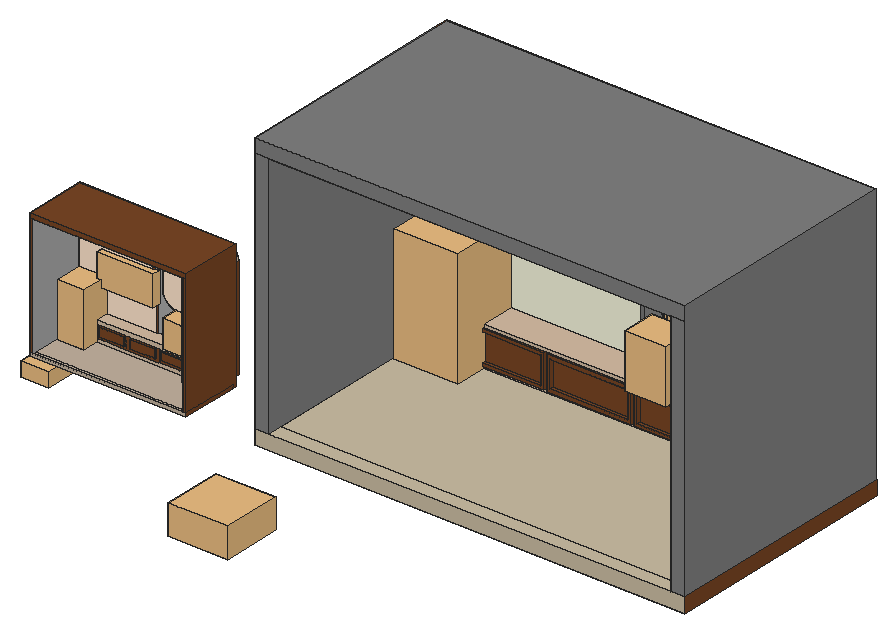
# SketchUp Ruby script. Lengths in inches.
U = 1.inch
M = Sketchup.active_model
def pt(a) = Geom::Point3d.new(a.map { |v| v * U })
def face(e, loops, mat)
  f = e.add_face(loops[0].map { |a| pt(a) })
  loops[1..].each { |l| e.add_face(l.map { |a| pt(a) }).erase! }
  f.material = f.back_material = mat if mat
  f
end
# faces: each face lists its corners as indices into pts; further lists are holes
def faces(e, pts, list, mat = nil) = list.each { |f| face(e, (f[0].is_a?(Array) ? f : [f]).map { |l| l.map { |i| pts[i] } }, mat) }
# xy, xz, yz: faces in a plane at the given z, y or x. An outline is a flat list of corners, or four numbers for a rectangle; further outlines are holes
def ring(l) = l.size == 4 ? [[l[0], l[1]], [l[2], l[1]], [l[2], l[3]], [l[0], l[3]]] : l.each_slice(2).to_a
def flat(e, list, mat, &to3) = list.each { |f| face(e, (f[0].is_a?(Array) ? f : [f]).map { |l| ring(l).map { |u, v| to3.(u, v) } }, mat) }
def xy(e, z, list, mat = nil) = flat(e, list, mat) { |x, y| [x, y, z] }
def xz(e, y, list, mat = nil) = flat(e, list, mat) { |x, z| [x, y, z] }
def yz(e, x, list, mat = nil) = flat(e, list, mat) { |y, z| [x, y, z] }
def lines(e, pts, list) = list.each { |a, b| e.add_line(pt(pts[a]), pt(pts[b])) }
# prism: a flat outline (further loops are holes) pulled along v
def prism(e, loops, v, mat = nil)
  f = face(e, loops, mat); d = Geom::Vector3d.new(v.map { |x| x * U })
  f.pushpull(f.normal.samedirection?(d) ? d.length : -d.length)
end
def box(e, o, s, mat = nil) = prism(e, [[o, [o[0] + s[0], o[1], o[2]], [o[0] + s[0], o[1] + s[1], o[2]], [o[0], o[1] + s[1], o[2]]]], [0, 0, s[2]], mat)
def at(x, y, z, deg = 0) = Geom::Transformation.translation(pt([x, y, z])) * Geom::Transformation.rotation(ORIGIN, Z_AXIS, deg.degrees)
def axes(o, x, y, z) = Geom::Transformation.new([*x, 0, *y, 0, *z, 0, *pt(o).to_a, 1])
def part(name) = M.definitions.add(name)
# library, detail: a bought-in or finely detailed component or shape, given as its bounding box
def library(name, o, s) = part(name).tap { |d| box(d.entities, o, s) }
def detail(e, o, s) = box(e.add_group.entities, o, s)
def put(e, d, t, mat = nil) = e.add_instance(d, t).tap { |i| i.material = mat if mat }
def group(e, t, mat = nil) = e.add_group.tap { |g| g.transformation = t; g.material = mat if mat }.entities
root = M.entities
M.materials.add("[0049_Beige]").color = [245, 245, 220]
M.materials.add("[0131_Silver]").color = [192, 192, 192]
M.materials.add("[0132_LightGray]").color = [169, 169, 169]
M.materials.add("[0133_Gray]").color = [128, 128, 128]
M.materials.add("[Color C01]").color = [255, 229, 204]
M.materials.add("[Concrete Tile]").color = [203, 190, 164]
M.materials.add("[Formica Laminate Light]").color = [213, 189, 164]
M.materials.add("[Tile Large Brown]").color = [195, 178, 159]
M.materials.add("[Wood Veneer 01]").color = [120, 70, 37]
c1 = library("Vase 296 007 001",[-21.53,-18.1,-0.16],[43.06,36.19,57.09])
c2 = library("False Aralia 002",[-20.33,-19.19,0],[40.48,38.23,49.87])
c3 = library("Clock Wall 005",[-16.6,-6.65,-37.13],[33.15,6.65,38.31])
c4 = library("Television screen",[0,1.41,1.14],[35.92,0.28,20.21])
c5 = library("Spot Light",[-5.1,-5.1,-11.05],[10.2,10.2,11.05])
c6 = library("Dome Light",[-12,-12,0],[24,24,12])
c7 = part("Group16\#1")
p = [[0,0,0],[0,0,-66.45],[-11.6,0,-66.45],[75.53,-139.58,0],[-75.53,-139.58,0],[75.53,139.58,0],
  [75.53,0,0],[-75.53,139.58,0],[11.6,0,-66.45],[-75.53,0,0],[0,0,-107.56]]
lines(c7.entities,p,[[0,1],[1,2],[3,4],[5,6],[7,5],[1,8],[9,0],[0,6],[8,10],[4,9],[6,3],[2,10],
  [9,7]])
c8 = part("Rectangle Light")
put(c8.entities,c7,at(0,0,0))
c9 = library("Omni Light",[-12,-12,-12],[24,24,24])
c10 = library("Omni Light\#1",[-12,-12,-12],[24,24,24])
c11 = library("Omni Light\#2",[-12,-12,-12],[24,24,24])
c12 = library("Omni Light\#3",[-12,-12,-12],[24,24,24])
c13 = library("Omni Light\#4",[-12,-12,-12],[24,24,24])
c14 = library("Omni Light\#5",[-12,-12,-12],[24,24,24])
c15 = library("Omni Light\#6",[-12,-12,-12],[24,24,24])
c16 = library("Omni Light\#7",[-12,-12,-12],[24,24,24])
c17 = library("Omni Light\#8",[-12,-12,-12],[24,24,24])
c18 = library("Omni Light\#9",[-12,-12,-12],[24,24,24])
c19 = library("Omni Light\#10",[-12,-12,-12],[24,24,24])
c20 = library("Omni Light\#11",[-12,-12,-12],[24,24,24])
c21 = library("Omni Light\#12",[-12,-12,-12],[24,24,24])
c22 = library("Omni Light\#13",[-12,-12,-12],[24,24,24])
c23 = library("Omni Light\#14",[-12,-12,-12],[24,24,24])
c24 = library("Omni Light\#15",[-12,-12,-12],[24,24,24])
c25 = library("Omni Light\#16",[-12,-12,-12],[24,24,24])
c26 = library("Omni Light\#17",[-12,-12,-12],[24,24,24])
c27 = library("Omni Light\#18",[-12,-12,-12],[24,24,24])
c28 = library("Omni Light\#19",[-12,-12,-12],[24,24,24])
c29 = library("Omni Light\#20",[-12,-12,-12],[24,24,24])
c30 = library("Omni Light\#21",[-12,-12,-12],[24,24,24])
c31 = library("Omni Light\#22",[-12,-12,-12],[24,24,24])
c32 = library("Omni Light\#23",[-12,-12,-12],[24,24,24])
c33 = library("Omni Light\#24",[-12,-12,-12],[24,24,24])
c34 = library("Omni Light\#25",[-12,-12,-12],[24,24,24])
c35 = library("Dome Light\#1",[-12,-12,0],[24,24,12])
c36 = library("Group\#5",[0,0,0],[151,81.0625,281.6875])
c37 = library("Group\#7",[0,0,0],[106.53,4.9375,165.91])
xy(root,0,[[472.95,0,1373.83,501.25]],"[Wood Veneer 01]")
xy(root,7.3125,[[7.02,1.49,320.41,8.52],[7.02,8.52,320.41,8.52,320.41,78.66,314.79,78.66,314.79,154.47,262.16,154.47,262.16,78.66,256.35,78.66,256.35,124.34,256.15,124.34,256.15,95.03,64.79,95.03,63.9,95.09,63.02,95.26,62.18,95.55,61.375,95.95,60.63,96.44,59.96,97.03,59.37,97.7,58.875,98.45,58.48,99.25,58.19,100.09,58.02,100.97,57.96,101.86,57.96,121.47,7.02,121.47]],"[Tile Large Brown]")
xy(root,19.25,[[68.6,95.03,122.4,97.28],[134.41,95.03,188.21,97.28],[199.24,95.03,253.04,97.28]],"[Wood Veneer 01]")
xy(root,19.89,[[199.875,95.03,252.4,97.28]],"[Wood Veneer 01]")
xy(root,20.02,[[135.18,95.03,187.44,97.28]],"[Wood Veneer 01]")
xy(root,20.04,[[69.39,95.03,121.61,97.28]],"[Wood Veneer 01]")
xy(root,30.1875,[[472.95,0,1373.83,0,1373.83,471.59,1344.17,471.59,1344.17,29.66,502.62,29.66,502.62,471.59,472.95,471.59],[502.62,29.66,1344.17,29.66,1344.17,471.59,1342.17,471.59,1342.17,390.53,1323.54,390.53,1323.54,471.59,1312.73,471.59,1312.73,390.53,1306.5,390.53,1306.5,471.59,1295.58,471.59,1295.58,386.34,1290.74,386.34,1290.74,471.59,1183.92,471.59,1183.92,386.34,1179.08,386.34,1179.08,471.59,1168.14,471.59,1168.14,390.53,1161.92,390.53,1161.92,471.59,1147.79,471.59,1147.79,390.53,1126.36,390.53,1126.36,392.15,599.34,392.15,599.34,471.59,502.62,471.59]],"[Concrete Tile]")
xy(root,30.1875,[[599.34,392.15,1126.36,471.59]],"[Wood Veneer 01]")
xy(root,36.08,[[605.24,387.03,768.36,392.15],[774.36,387.03,951.86,392.15],[957.86,387.03,1120.46,392.15]],"[Wood Veneer 01]")
xy(root,37.21,[[69.39,95.03,121.61,97.28]],"[Wood Veneer 01]")
xy(root,37.23,[[135.18,95.03,187.44,97.28]],"[Wood Veneer 01]")
xy(root,37.36,[[199.875,95.03,252.4,97.28]],"[Wood Veneer 01]")
xy(root,38,[[68.6,95.03,122.4,97.28],[134.41,95.03,188.21,97.28],[199.24,95.03,253.04,97.28]],"[Wood Veneer 01]")
xy(root,41.83,[[610.98,387.03,762.62,395.59]],"[Wood Veneer 01]")
xy(root,42.55,[[964.33,387.03,1113.99,394.15]],"[Wood Veneer 01]")
xy(root,43.18,[[781.45,387.03,944.77,394.15]],"[Wood Veneer 01]")
xy(root,50.1875,[[64.79,95.03,65.54,95.03,65.54,95.87,64.65,95.92,63.78,96.1,62.93,96.38,62.13,96.78,61.39,97.28,60.72,97.86,60.13,98.54,59.63,99.28,59.24,100.08,58.95,100.92,58.78,101.8,58.72,102.69,57.96,102.69,57.96,101.86,58.02,100.97,58.19,100.09,58.48,99.25,58.875,98.45,59.37,97.7,59.96,97.03,60.63,96.44,61.375,95.95,62.18,95.55,63.02,95.26,63.9,95.09]],"[0131_Silver]")
xy(root,50.1875,[[65.54,95.03,256.15,95.03,256.15,124.34,170.4,124.34,170.4,121.47,57.96,121.47,57.96,102.69,58.72,102.69,58.78,101.8,58.95,100.92,59.24,100.08,59.63,99.28,60.13,98.54,60.72,97.86,61.39,97.28,62.13,96.78,62.93,96.38,63.78,96.1,64.65,95.92,65.54,95.87]],"[Formica Laminate Light]")
xy(root,56.81,[[1183.92,386.34,1290.74,387.61],[1183.92,387.61,1290.74,466.75],[1183.92,466.75,1290.74,471.59]],"[Wood Veneer 01]")
xy(root,61.79,[[1184.07,386.34,1290.6,388.34]],"[Wood Veneer 01]")
xy(root,99.69,[[781.45,387.03,944.77,394.15]],"[Wood Veneer 01]")
xy(root,100.3125,[[964.33,387.03,1113.99,394.15]],"[Wood Veneer 01]")
xy(root,101.04,[[610.98,387.03,762.62,395.59]],"[Wood Veneer 01]")
xy(root,106.78,[[605.24,387.03,768.36,392.15],[774.36,387.03,951.86,392.15],[957.86,387.03,1120.46,392.15]],"[Wood Veneer 01]")
xy(root,112.68,[[599.34,392.15,1126.36,392.15,1126.36,471.59,910.87,471.59,910.87,463.9,599.34,463.9]],"[Formica Laminate Light]")
xy(root,112.68,[[599.34,463.9,910.87,471.59]],"[Wood Veneer 01]")
xy(root,227.7,[[1184.07,386.34,1290.6,388.34]],"[Wood Veneer 01]")
xy(root,232.6875,[[1179.08,386.34,1295.58,471.59]],"[Wood Veneer 01]")
xy(root,259.9375,[[[7.02,1.49,7.02,124.34,181.32,124.34,181.32,122.16,242.7,122.16,242.7,124.34,256.35,124.34,256.35,78.66,320.41,78.66,320.41,1.49],[167.78,30.28,172.11,30.85,176.14,32.52,179.6,35.18,182.26,38.64,183.93,42.67,184.5,47,183.93,51.32,182.26,55.36,179.6,58.82,176.14,61.47,172.11,63.14,167.78,63.71,163.46,63.14,159.42,61.47,155.96,58.82,153.31,55.36,151.64,51.32,151.07,47,151.64,42.67,153.31,38.64,155.96,35.18,159.42,32.52,163.46,30.85],[71.01,30.28,75.34,30.85,79.37,32.52,82.83,35.18,85.49,38.64,87.16,42.67,87.73,47,87.16,51.32,85.49,55.36,82.83,58.82,79.37,61.47,75.34,63.14,71.01,63.71,66.69,63.14,62.65,61.47,59.19,58.82,56.54,55.36,54.87,51.32,54.3,47,54.87,42.67,56.54,38.64,59.19,35.18,62.65,32.52,66.69,30.85],[260.125,30.28,264.45,30.85,268.48,32.52,271.95,35.18,274.6,38.64,276.27,42.67,276.84,47,276.27,51.32,274.6,55.36,271.95,58.82,268.48,61.47,264.45,63.14,260.125,63.71,255.8,63.14,251.77,61.47,248.31,58.82,245.65,55.36,243.98,51.32,243.41,47,243.98,42.67,245.65,38.64,248.31,35.18,251.77,32.52,255.8,30.85]],[[71.01,30.28,66.69,30.85,62.65,32.52,59.19,35.18,56.54,38.64,54.87,42.67,54.3,47,54.87,51.32,56.54,55.36,59.19,58.82,62.65,61.47,66.69,63.14,71.01,63.71,75.34,63.14,79.37,61.47,82.83,58.82,85.49,55.36,87.16,51.32,87.73,47,87.16,42.67,85.49,38.64,82.83,35.18,79.37,32.52,75.34,30.85],[71.01,33.59,74.48,34.05,77.71,35.39,80.49,37.52,82.62,40.3,83.96,43.53,84.42,47,83.96,50.47,82.62,53.7,80.49,56.48,77.71,58.61,74.48,59.95,71.01,60.4,67.54,59.95,64.31,58.61,61.53,56.48,59.4,53.7,58.0625,50.47,57.61,47,58.0625,43.53,59.4,40.3,61.53,37.52,64.31,35.39,67.54,34.05]],[[167.78,30.28,163.46,30.85,159.42,32.52,155.96,35.18,153.31,38.64,151.64,42.67,151.07,47,151.64,51.32,153.31,55.36,155.96,58.82,159.42,61.47,163.46,63.14,167.78,63.71,172.11,63.14,176.14,61.47,179.6,58.82,182.26,55.36,183.93,51.32,184.5,47,183.93,42.67,182.26,38.64,179.6,35.18,176.14,32.52,172.11,30.85],[167.78,33.15,171.37,33.62,174.71,35.01,177.57,37.21,179.77,40.07,181.16,43.41,181.63,47,181.16,50.58,179.77,53.92,177.57,56.79,174.71,58.99,171.37,60.375,167.78,60.85,164.2,60.375,160.86,58.99,157.99,56.79,155.79,53.92,154.41,50.58,153.93,47,154.41,43.41,155.79,40.07,157.99,37.21,160.86,35.01,164.2,33.62]],[[260.125,30.28,255.8,30.85,251.77,32.52,248.31,35.18,245.65,38.64,243.98,42.67,243.41,47,243.98,51.32,245.65,55.36,248.31,58.82,251.77,61.47,255.8,63.14,260.125,63.71,264.45,63.14,268.48,61.47,271.95,58.82,274.6,55.36,276.27,51.32,276.84,47,276.27,42.67,274.6,38.64,271.95,35.18,268.48,32.52,264.45,30.85],[260.125,32.92,263.77,33.4,267.17,34.8,270.08,37.04,272.32,39.96,273.73,43.35,274.21,47,273.73,50.64,272.32,54.04,270.08,56.95,267.17,59.19,263.77,60.6,260.125,61.08,256.48,60.6,253.09,59.19,250.17,56.95,247.93,54.04,246.53,50.64,246.05,47,246.53,43.35,247.93,39.96,250.17,37.04,253.09,34.8,256.48,33.4]]],"[0132_LightGray]")
xy(root,262.5625,[[260.125,32.92,256.48,33.4,253.09,34.8,250.17,37.04,247.93,39.96,246.53,43.35,246.05,47,246.53,50.64,247.93,54.04,250.17,56.95,253.09,59.19,256.48,60.6,260.125,61.08,263.77,60.6,267.17,59.19,270.08,56.95,272.32,54.04,273.73,50.64,274.21,47,273.73,43.35,272.32,39.96,270.08,37.04,267.17,34.8,263.77,33.4]],"[0132_LightGray]")
xy(root,262.6875,[[167.78,33.15,164.2,33.62,160.86,35.01,157.99,37.21,155.79,40.07,154.41,43.41,153.93,47,154.41,50.58,155.79,53.92,157.99,56.79,160.86,58.99,164.2,60.375,167.78,60.85,171.37,60.375,174.71,58.99,177.57,56.79,179.77,53.92,181.16,50.58,181.63,47,181.16,43.41,179.77,40.07,177.57,37.21,174.71,35.01,171.37,33.62]],"[0132_LightGray]")
xy(root,263.25,[[71.01,33.59,67.54,34.05,64.31,35.39,61.53,37.52,59.4,40.3,58.0625,43.53,57.61,47,58.0625,50.47,59.4,53.7,61.53,56.48,64.31,58.61,67.54,59.95,71.01,60.4,74.48,59.95,77.71,58.61,80.49,56.48,82.62,53.7,83.96,50.47,84.42,47,83.96,43.53,82.62,40.3,80.49,37.52,77.71,35.39,74.48,34.05]],"[0132_LightGray]")
xy(root,268.9375,[[0,1.49,327.4375,131.37]],"[Wood Veneer 01]")
xy(root,547.5625,[[1126.36,390.53,1342.17,471.59]],"[Wood Veneer 01]")
xz(root,0,[[472.95,0,1373.83,30.1875]],"[Concrete Tile]")
xz(root,1.49,[[0,0,327.4375,7.3125]],"[Tile Large Brown]")
xz(root,1.49,[[0,7.3125,7.02,259.9375],[320.41,7.3125,327.4375,259.9375],[0,259.9375,327.4375,268.9375]],"[Wood Veneer 01]")
xz(root,78.66,[[256.35,7.3125,262.16,7.3125,262.16,222.3125,263.06,229.12,265.6875,235.47,269.87,240.92,275.32,245.1,281.67,247.73,288.48,248.625,295.29,247.73,301.63,245.1,307.08,240.92,311.26,235.47,313.89,229.12,314.79,222.3125,314.79,7.3125,320.41,7.3125,320.41,259.9375,256.35,259.9375]],"[Formica Laminate Light]")
xz(root,95.03,[[[64.79,7.3125,256.15,7.3125,256.15,50.1875,64.79,50.1875,64.79,41.8125,126.21,41.8125,126.21,15.4375,64.79,15.4375],[126.71,15.4375,195.46,41.8125],[195.96,15.4375,255.65,41.8125]]],"[Formica Laminate Light]")
xz(root,95.03,[[[64.79,15.4375,126.21,41.8125],[68.6,19.25,122.4,38]],[[126.71,15.4375,195.46,41.8125],[134.41,19.25,188.21,38]],[[195.96,15.4375,255.65,41.8125],[199.24,19.25,253.04,38]],[199.875,19.89,252.4,37.36],[135.18,20.02,187.44,37.23],
  [69.39,20.04,121.61,37.21]],"[Wood Veneer 01]")
xz(root,97.28,[[[68.6,19.25,122.4,38],[69.39,20.04,121.61,37.21]],[[134.41,19.25,188.21,38],[135.18,20.02,187.44,37.23]],[[199.24,19.25,253.04,38],[199.875,19.89,252.4,37.36]]],"[0131_Silver]")
xz(root,124.34,[[256.15,7.3125,256.35,7.3125,256.35,259.9375,242.7,259.9375,242.7,136.85,241.65,128.91,238.59,121.51,233.71,115.15,227.35,110.28,219.95,107.21,212.01,106.16,204.07,107.21,196.67,110.28,190.31,115.15,185.43,121.51,182.37,128.91,181.32,136.85,181.32,259.9375,7.02,259.9375,7.02,203.375,106.35,203.375,114.93,202.8,123.36,201.08,131.48,198.24,139.15,194.35,146.23,189.46,152.59,183.67,158.11,177.08,162.71,169.8125,166.29,161.99,168.79,153.76,170.17,145.27,170.4,136.68,170.4,50.1875,256.15,50.1875]],"[0132_LightGray]")
xz(root,131.37,[[0,0,327.4375,268.9375]],"[Formica Laminate Light]")
xz(root,154.47,[[262.16,7.3125,314.79,7.3125,314.79,222.3125,313.89,229.12,311.26,235.47,307.08,240.92,301.63,245.1,295.29,247.73,288.48,248.625,281.67,247.73,275.32,245.1,269.87,240.92,265.6875,235.47,263.06,229.12,262.16,222.3125]],"[Wood Veneer 01]")
xz(root,386.34,[[[1179.08,30.1875,1183.92,30.1875,1183.92,56.81,1290.74,56.81,1290.74,30.1875,1295.58,30.1875,1295.58,232.6875,1179.08,232.6875],[1184.07,61.79,1290.6,227.7]]],"[Wood Veneer 01]")
xz(root,387.03,[[[605.24,36.08,768.36,106.78],[610.98,41.83,762.62,101.04]],[[774.36,36.08,951.86,106.78],[781.45,43.18,944.77,99.69]],[[957.86,36.08,1120.46,106.78],[964.33,42.55,1113.99,100.3125]]],"[Wood Veneer 01]")
xz(root,390.53,[[1126.36,30.1875,1147.79,30.1875,1147.79,444.6875,1152.17,466.13,1161.7,485.83,1175.79,502.58,1193.57,515.34,1213.95,523.33,1235.67,526.04,1257.38,523.33,1277.76,515.34,1295.54,502.58,1309.63,485.83,1319.16,466.13,1323.54,444.6875,1323.54,30.1875,1342.17,30.1875,1342.17,547.5625,1126.36,547.5625]],"[Formica Laminate Light]")
xz(root,392.15,[[[599.34,30.1875,1126.36,112.68],[605.24,36.08,1120.46,106.78]],[768.36,36.08,774.36,106.78],[951.86,36.08,957.86,106.78]],"[Formica Laminate Light]")
xz(root,394.15,[[964.33,42.55,1113.99,100.3125],[781.45,43.18,944.77,99.69]],"[Wood Veneer 01]")
xz(root,395.59,[[610.98,41.83,762.62,101.04]],"[Wood Veneer 01]")
xz(root,455.26,[[1039.84,192.87,1059.39,195.45,1077.6,202.99,1093.25,214.99,1105.25,230.64,1112.8,248.85,1115.37,268.4,1115.37,547.5625,964.31,547.5625,964.31,268.4,966.88,248.85,974.43,230.64,986.43,214.99,1002.07,202.99,1020.29,195.45]],"[0049_Beige]")
xz(root,462.88,[[1040.15,192.87,1020.6,195.45,1002.38,202.99,986.74,214.99,974.74,230.64,967.19,248.85,964.62,268.4,1115.68,268.4,1113.11,248.85,1105.5625,230.64,1093.56,214.99,1077.92,202.99,1059.7,195.45],[964.62,268.4,964.31,547.5625,1115.37,547.5625,1115.68,268.4]],"[Wood Veneer 01]")
xz(root,471.59,[[599.34,30.1875,1126.36,112.68],[1183.92,30.1875,1290.74,56.81]],"[Wood Veneer 01]")
yz(root,0,[[1.49,0,124.34,7.3125],[124.34,0,124.34,7.3125,1.49,7.3125,1.49,268.9375,131.37,268.9375,131.37,0]],"[Wood Veneer 01]")
yz(root,7.02,[[1.49,7.3125,124.34,259.9375]],"[0132_LightGray]")
yz(root,57.96,[[101.86,7.3125,121.47,50.1875]],"[Formica Laminate Light]")
yz(root,68.6,[[95.03,19.25,97.28,38]],"[Wood Veneer 01]")
yz(root,69.39,[[95.03,20.04,97.28,37.21]],"[Wood Veneer 01]")
yz(root,121.61,[[95.03,20.04,97.28,37.21]],"[Wood Veneer 01]")
yz(root,122.4,[[95.03,19.25,97.28,38]],"[Wood Veneer 01]")
yz(root,134.41,[[95.03,19.25,97.28,38]],"[Wood Veneer 01]")
yz(root,135.18,[[95.03,20.02,97.28,37.23]],"[Wood Veneer 01]")
yz(root,181.32,[[122.16,136.85,124.34,259.9375]],"[Wood Veneer 01]")
yz(root,187.44,[[95.03,20.02,97.28,37.23]],"[Wood Veneer 01]")
yz(root,188.21,[[95.03,19.25,97.28,38]],"[Wood Veneer 01]")
yz(root,199.24,[[95.03,19.25,97.28,38]],"[Wood Veneer 01]")
yz(root,199.875,[[95.03,19.89,97.28,37.36]],"[Wood Veneer 01]")
yz(root,242.7,[[122.16,136.85,124.34,259.9375]],"[Wood Veneer 01]")
yz(root,252.4,[[95.03,19.89,97.28,37.36]],"[Wood Veneer 01]")
yz(root,253.04,[[95.03,19.25,97.28,38]],"[Wood Veneer 01]")
yz(root,256.15,[[95.03,7.3125,124.34,50.1875]],"[Wood Veneer 01]")
yz(root,256.35,[[78.66,7.3125,124.34,259.9375]],"[Formica Laminate Light]")
yz(root,262.16,[[78.66,7.3125,131.37,222.3125]],"[Formica Laminate Light]")
yz(root,262.16,[[131.37,7.3125,154.47,222.3125]],"[Wood Veneer 01]")
yz(root,314.79,[[78.66,7.3125,131.37,222.3125]],"[Formica Laminate Light]")
yz(root,314.79,[[131.37,7.3125,154.47,222.3125]],"[Wood Veneer 01]")
yz(root,320.41,[[1.49,7.3125,78.66,259.9375]],"[0132_LightGray]")
yz(root,327.4375,[[1.49,0,124.34,7.3125],[124.34,0,131.37,0,131.37,268.9375,1.49,268.9375,1.49,7.3125,124.34,7.3125]],"[Wood Veneer 01]")
yz(root,472.95,[[0,0,501.25,30.1875],[471.59,30.1875,501.25,576.6875]],"[Wood Veneer 01]")
yz(root,599.34,[[392.15,30.1875,471.59,112.68]],"[Wood Veneer 01]")
yz(root,605.24,[[387.03,36.08,392.15,106.78]],"[Wood Veneer 01]")
yz(root,610.98,[[387.03,41.83,395.59,101.04]],"[Wood Veneer 01]")
yz(root,762.62,[[387.03,41.83,395.59,101.04]],"[Wood Veneer 01]")
yz(root,768.36,[[387.03,36.08,392.15,106.78]],"[Wood Veneer 01]")
yz(root,774.36,[[387.03,36.08,392.15,106.78]],"[Wood Veneer 01]")
yz(root,781.45,[[387.03,43.18,394.15,99.69]],"[Wood Veneer 01]")
yz(root,944.77,[[387.03,43.18,394.15,99.69]],"[Wood Veneer 01]")
yz(root,951.86,[[387.03,36.08,392.15,106.78]],"[Wood Veneer 01]")
yz(root,957.86,[[387.03,36.08,392.15,106.78]],"[Wood Veneer 01]")
yz(root,964.33,[[387.03,42.55,394.15,100.3125]],"[Wood Veneer 01]")
yz(root,1113.99,[[387.03,42.55,394.15,100.3125]],"[Wood Veneer 01]")
yz(root,1120.46,[[387.03,36.08,392.15,106.78]],"[Wood Veneer 01]")
yz(root,1126.36,[[390.53,112.68,471.59,547.5625]],"[Formica Laminate Light]")
yz(root,1126.36,[[390.53,30.1875,392.15,112.68]],"[Wood Veneer 01]")
yz(root,1147.79,[[390.53,30.1875,471.59,444.6875]],"[Formica Laminate Light]")
yz(root,1179.08,[[386.34,30.1875,471.59,232.6875]],"[Wood Veneer 01]")
yz(root,1183.92,[[386.34,30.1875,387.61,56.81],[387.61,30.1875,466.75,56.81],[466.75,30.1875,471.59,56.81]],"[Wood Veneer 01]")
yz(root,1184.07,[[386.34,61.79,388.34,227.7]],"[Wood Veneer 01]")
yz(root,1290.6,[[386.34,61.79,388.34,227.7]],"[Wood Veneer 01]")
yz(root,1290.74,[[386.34,30.1875,387.61,56.81],[387.61,30.1875,466.75,56.81],[466.75,30.1875,471.59,56.81]],"[Wood Veneer 01]")
yz(root,1295.58,[[386.34,30.1875,471.59,232.6875]],"[Wood Veneer 01]")
yz(root,1323.54,[[390.53,30.1875,471.59,444.6875]],"[Formica Laminate Light]")
yz(root,1342.17,[[390.53,30.1875,471.59,547.5625]],"[Wood Veneer 01]")
yz(root,1373.83,[[0,0,501.25,30.1875]],"[Wood Veneer 01]")
p = [[64.79,95.03,50.1875],[63.9,95.09,50.1875],[63.9,95.09,7.3125],[64.79,95.03,7.3125],[64.79,95.03,15.4375],[64.79,95.03,41.8125],
  [63.02,95.26,50.1875],[63.02,95.26,7.3125],[62.18,95.55,50.1875],[62.18,95.55,7.3125],[61.375,95.95,50.1875],[61.375,95.95,7.3125],
  [60.63,96.44,50.1875],[60.63,96.44,7.3125],[59.96,97.03,50.1875],[59.96,97.03,7.3125],[59.37,97.7,50.1875],[59.37,97.7,7.3125],
  [58.875,98.45,50.1875],[58.875,98.45,7.3125],[58.48,99.25,50.1875],[58.48,99.25,7.3125],[58.19,100.09,50.1875],[58.19,100.09,7.3125],
  [58.02,100.97,50.1875],[58.02,100.97,7.3125],[57.96,101.86,50.1875],[57.96,101.86,7.3125],[204.07,124.34,107.21],[212.01,124.34,106.16],
  [212.01,122.16,106.16],[204.07,122.16,107.21],[219.95,124.34,107.21],[219.95,122.16,107.21],[196.67,124.34,110.28],[196.67,122.16,110.28],
  [227.35,124.34,110.28],[227.35,122.16,110.28],[190.31,124.34,115.15],[190.31,122.16,115.15],[233.71,124.34,115.15],[233.71,122.16,115.15],
  [185.43,124.34,121.51],[185.43,122.16,121.51],[238.59,124.34,121.51],[238.59,122.16,121.51],[182.37,124.34,128.91],[182.37,122.16,128.91],
  [241.65,124.34,128.91],[241.65,122.16,128.91],[181.32,124.34,136.85],[181.32,122.16,136.85],[242.7,124.34,136.85],[242.7,122.16,136.85],
  [1020.6,462.88,195.45],[1040.15,462.88,192.87],[1039.84,455.26,192.87],[1020.29,455.26,195.45],[1059.7,462.88,195.45],[1059.39,455.26,195.45],
  [1002.38,462.88,202.99],[1002.07,455.26,202.99],[1077.92,462.88,202.99],[1077.6,455.26,202.99],[986.74,462.88,214.99],[986.43,455.26,214.99],
  [1093.56,462.88,214.99],[1093.25,455.26,214.99],[974.43,455.26,230.64],[974.74,462.88,230.64],[1105.5625,462.88,230.64],[1105.25,455.26,230.64],
  [263.06,78.66,229.12],[262.16,78.66,222.3125],[262.16,131.37,222.3125],[262.16,154.47,222.3125],[263.06,154.47,229.12],[314.79,78.66,222.3125],
  [313.89,78.66,229.12],[313.89,154.47,229.12],[314.79,154.47,222.3125],[314.79,131.37,222.3125],[265.6875,78.66,235.47],[265.6875,154.47,235.47],
  [311.26,78.66,235.47],[311.26,154.47,235.47],[966.88,455.26,248.85],[967.19,462.88,248.85],[1113.11,462.88,248.85],[1112.8,455.26,248.85],
  [269.87,78.66,240.92],[269.87,154.47,240.92],[307.08,78.66,240.92],[307.08,154.47,240.92],[275.32,78.66,245.1],[275.32,154.47,245.1],
  [301.63,78.66,245.1],[301.63,154.47,245.1],[281.67,78.66,247.73],[281.67,154.47,247.73],[295.29,78.66,247.73],[295.29,154.47,247.73],
  [288.48,78.66,248.625],[288.48,154.47,248.625],[964.31,455.26,268.4],[964.62,462.88,268.4],[1115.68,462.88,268.4],[1115.37,455.26,268.4],
  [260.125,32.92,259.9375],[256.48,33.4,259.9375],[256.48,33.4,262.5625],[260.125,32.92,262.5625],[263.77,33.4,259.9375],[263.77,33.4,262.5625],
  [167.78,33.15,259.9375],[164.2,33.62,259.9375],[164.2,33.62,262.6875],[167.78,33.15,262.6875],[171.37,33.62,259.9375],[171.37,33.62,262.6875],
  [253.09,34.8,259.9375],[253.09,34.8,262.5625],[267.17,34.8,259.9375],[267.17,34.8,262.5625],[71.01,33.59,259.9375],[67.54,34.05,259.9375],
  [67.54,34.05,263.25],[71.01,33.59,263.25],[74.48,34.05,259.9375],[74.48,34.05,263.25],[160.86,35.01,259.9375],[160.86,35.01,262.6875],
  [174.71,35.01,259.9375],[174.71,35.01,262.6875],[64.31,35.39,259.9375],[64.31,35.39,263.25],[77.71,35.39,259.9375],[77.71,35.39,263.25],
  [250.17,37.04,259.9375],[250.17,37.04,262.5625],[270.08,37.04,259.9375],[270.08,37.04,262.5625],[157.99,37.21,259.9375],[157.99,37.21,262.6875],
  [177.57,37.21,259.9375],[177.57,37.21,262.6875],[61.53,37.52,259.9375],[61.53,37.52,263.25],[80.49,37.52,259.9375],[80.49,37.52,263.25],
  [247.93,39.96,259.9375],[247.93,39.96,262.5625],[272.32,39.96,259.9375],[272.32,39.96,262.5625],[155.79,40.07,259.9375],[155.79,40.07,262.6875],
  [179.77,40.07,259.9375],[179.77,40.07,262.6875],[59.4,40.3,259.9375],[59.4,40.3,263.25],[82.62,40.3,259.9375],[82.62,40.3,263.25],
  [246.53,43.35,259.9375],[246.53,43.35,262.5625],[273.73,43.35,259.9375],[273.73,43.35,262.5625],[154.41,43.41,259.9375],[154.41,43.41,262.6875],
  [181.16,43.41,259.9375],[181.16,43.41,262.6875],[58.0625,43.53,259.9375],[58.0625,43.53,263.25],[83.96,43.53,259.9375],[83.96,43.53,263.25],
  [153.93,47,259.9375],[153.93,47,262.6875],[181.63,47,259.9375],[181.63,47,262.6875],[246.05,47,259.9375],[246.05,47,262.5625],
  [274.21,47,259.9375],[274.21,47,262.5625],[57.61,47,259.9375],[57.61,47,263.25],[84.42,47,259.9375],[84.42,47,263.25],
  [58.0625,50.47,259.9375],[58.0625,50.47,263.25],[83.96,50.47,259.9375],[83.96,50.47,263.25],[154.41,50.58,259.9375],[154.41,50.58,262.6875],
  [181.16,50.58,259.9375],[181.16,50.58,262.6875],[246.53,50.64,259.9375],[246.53,50.64,262.5625],[273.73,50.64,259.9375],[273.73,50.64,262.5625],
  [59.4,53.7,259.9375],[59.4,53.7,263.25],[82.62,53.7,259.9375],[82.62,53.7,263.25],[155.79,53.92,259.9375],[155.79,53.92,262.6875],
  [179.77,53.92,259.9375],[179.77,53.92,262.6875],[247.93,54.04,259.9375],[247.93,54.04,262.5625],[272.32,54.04,259.9375],[272.32,54.04,262.5625],
  [61.53,56.48,259.9375],[61.53,56.48,263.25],[80.49,56.48,259.9375],[80.49,56.48,263.25],[157.99,56.79,259.9375],[157.99,56.79,262.6875],
  [177.57,56.79,259.9375],[177.57,56.79,262.6875],[250.17,56.95,259.9375],[250.17,56.95,262.5625],[270.08,56.95,259.9375],[270.08,56.95,262.5625],
  [64.31,58.61,259.9375],[64.31,58.61,263.25],[77.71,58.61,259.9375],[77.71,58.61,263.25],[160.86,58.99,259.9375],[160.86,58.99,262.6875],
  [174.71,58.99,259.9375],[174.71,58.99,262.6875],[253.09,59.19,259.9375],[253.09,59.19,262.5625],[267.17,59.19,259.9375],[267.17,59.19,262.5625],
  [67.54,59.95,259.9375],[67.54,59.95,263.25],[74.48,59.95,259.9375],[74.48,59.95,263.25],[164.2,60.375,259.9375],[164.2,60.375,262.6875],
  [171.37,60.375,259.9375],[171.37,60.375,262.6875],[256.48,60.6,259.9375],[256.48,60.6,262.5625],[263.77,60.6,259.9375],[263.77,60.6,262.5625],
  [71.01,60.4,259.9375],[71.01,60.4,263.25],[167.78,60.85,259.9375],[167.78,60.85,262.6875],[260.125,61.08,259.9375],[260.125,61.08,262.5625],
  [964.31,455.26,547.5625],[964.31,462.88,547.5625],[1115.37,455.26,547.5625],[1115.37,462.88,547.5625],[1152.17,390.53,466.13],[1147.79,390.53,444.6875],
  [1147.79,471.59,444.6875],[1152.17,471.59,466.13],[1323.54,390.53,444.6875],[1319.16,390.53,466.13],[1319.16,471.59,466.13],[1323.54,471.59,444.6875],
  [1161.7,390.53,485.83],[1161.7,471.59,485.83],[1309.63,390.53,485.83],[1309.63,471.59,485.83],[1175.79,390.53,502.58],[1175.79,471.59,502.58],
  [1295.54,390.53,502.58],[1295.54,471.59,502.58],[1193.57,390.53,515.34],[1193.57,471.59,515.34],[1277.76,390.53,515.34],[1277.76,471.59,515.34],
  [1213.95,390.53,523.33],[1213.95,471.59,523.33],[1257.38,390.53,523.33],[1257.38,471.59,523.33],[1235.67,390.53,526.04],[1235.67,471.59,526.04],
  [242.7,124.34,71.8125],[242.7,124.34,69.48],[1161.92,471.59,30.1875],[1161.92,471.59,297.96],[1175.83,471.59,311.875],[1174.02,471.59,311.76],
  [1172.23,471.59,311.4],[1170.51,471.59,310.82],[1168.875,471.59,310.01],[1167.36,471.59,309],[1165.99,471.59,307.8],[1164.79,471.59,306.43],
  [1163.78,471.59,304.92],[1162.98,471.59,303.28],[1162.39,471.59,301.56],[1162.04,471.59,299.78],[1299.64,471.59,311.875],[1301.5625,471.59,311.74],
  [1303.45,471.59,311.32],[1305.25,471.59,310.63],[1306.93,471.59,309.7],[1308.46,471.59,308.52],[1309.81,471.59,307.14],[1310.9375,471.59,305.58],
  [1311.83,471.59,303.87],[1312.47,471.59,302.05],[1312.73,471.59,300.69],[1312.83,471.59,300.16],[1312.92,471.59,298.23],[1312.73,471.59,296.31],
  [1312.73,471.59,30.1875],[1168.14,471.59,297.96],[1168.14,471.59,30.1875],[1306.5,471.59,30.1875],[1306.5,471.59,296.625],[1306.68,471.59,298.4],
  [1306.63,471.59,299.42],[1306.62,471.59,299.51],[1306.44,471.59,300.42],[1306.1,471.59,301.39],[1305.63,471.59,302.3],[1305.03,471.59,303.125],
  [1304.32,471.59,303.86],[1303.51,471.59,304.48],[1302.61,471.59,304.97],[1301.66,471.59,305.34],[1300.66,471.59,305.56],[1299.42,471.59,305.65],
  [1175.83,471.59,305.65],[1174.83,471.59,305.58],[1173.84,471.59,305.39],[1172.89,471.59,305.0625],[1171.99,471.59,304.62],[1171.15,471.59,304.06],
  [1170.4,471.59,303.4],[1169.73,471.59,302.64],[1169.17,471.59,301.8],[1168.73,471.59,300.9],[1168.41,471.59,299.95],[1168.21,471.59,298.96],
  [1175.83,471.59,321.875],[1299.64,471.59,321.875]]
faces(root,p,[[0,1,2,3,4,5],[1,6,7,2],[6,8,9,7],[8,10,11,9],[10,12,13,11],[12,14,15,13],[14,16,17,15],[16,18,19,17],
  [18,20,21,19],[20,22,23,21],[22,24,25,23],[24,26,27,25]],"[0131_Silver]")
faces(root,p,[[28,29,30,31],[29,32,33,30],[34,28,31,35],[32,36,37,33],[38,34,35,39],[36,40,41,37],[42,38,39,43],[40,44,45,41],
  [46,42,43,47],[44,48,49,45],[50,46,47,51],[48,52,53,49],[54,55,56,57],[55,58,59,56],[60,54,57,61],[58,62,63,59],
  [64,60,61,65],[62,66,67,63],[65,68,69,64],[67,66,70,71],[68,86,87,69],[71,70,88,89],[86,104,105,87],[89,88,106,107],
  [253,105,252],[107,106,254],[255,254,106]],"[Wood Veneer 01]")
faces(root,p,[[72,73,74,75,76],[77,78,79,80,81],[82,72,76,83],[78,84,85,79],[90,82,83,91],[84,92,93,85],[94,90,91,95],[92,96,97,93],
  [98,94,95,99],[96,100,101,97],[102,98,99,103],[100,102,103,101],[256,257,258,259],[260,261,262,263],[264,256,259,265],[261,266,267,262],
  [268,264,265,269],[266,270,271,267],[272,268,269,273],[270,274,275,271],[276,272,273,277],[274,278,279,275],[280,276,277,281],[278,280,281,279]],"[Formica Laminate Light]")
faces(root,p,[[108,109,110,111],[112,108,111,113],[114,115,116,117],[118,114,117,119],[109,120,121,110],[122,112,113,123],[124,125,126,127],[128,124,127,129],
  [115,130,131,116],[132,118,119,133],[125,134,135,126],[136,128,129,137],[120,138,139,121],[140,122,123,141],[130,142,143,131],[144,132,133,145],
  [134,146,147,135],[148,136,137,149],[138,150,151,139],[152,140,141,153],[142,154,155,143],[156,144,145,157],[146,158,159,147],[160,148,149,161],
  [150,162,163,151],[164,152,153,165],[154,166,167,155],[168,156,157,169],[158,170,171,159],[172,160,161,173],[166,174,175,167],[176,168,169,177],
  [162,178,179,163],[180,164,165,181],[170,182,183,171],[184,172,173,185],[182,186,187,183],[188,184,185,189],[174,190,191,175],[192,176,177,193],
  [178,194,195,179],[196,180,181,197],[186,198,199,187],[200,188,189,201],[190,202,203,191],[204,192,193,205],[194,206,207,195],[208,196,197,209],
  [198,210,211,199],[212,200,201,213],[202,214,215,203],[216,204,205,217],[206,218,219,207],[220,208,209,221],[210,222,223,211],[224,212,213,225],
  [214,226,227,215],[228,216,217,229],[218,230,231,219],[232,220,221,233],[222,234,235,223],[236,224,225,237],[226,238,239,227],[240,228,229,241],
  [230,242,243,231],[244,232,233,245],[234,246,247,235],[246,236,237,247],[238,248,249,239],[248,240,241,249],[242,250,251,243],[250,244,245,251]],"[0132_LightGray]")
faces(root,p,[[104,252,105]],"[0049_Beige]")
lines(root,p,[[282,283],[284,285],[286,287],[287,288],[288,289],[289,290],[290,291],[291,292],[292,293],[293,294],[294,295],[295,296],
  [296,297],[297,285],[298,299],[299,300],[300,301],[301,302],[302,303],[303,304],[304,305],[305,306],[306,307],[307,308],
  [309,310],[310,311],[311,312],[308,309],[313,314],[315,316],[316,317],[317,318],[318,319],[319,320],[320,321],[321,322],
  [322,323],[323,324],[324,325],[325,326],[326,327],[327,328],[328,329],[329,330],[330,331],[331,332],[332,333],[333,334],
  [334,335],[335,336],[336,337],[337,338],[338,339],[339,340],[340,341],[341,313],[286,342],[298,343]])
detail(root,[1167.4,390.53,321.875],[141.62,81.06,22.1875])
put(root,c1,at(231.47,104.52,50.1875),"[Wood Veneer 01]")
put(root,c2,axes([29.94,96.35,7.3125],[1.74,0,0],[0,1.74,0],[0,0,2.2446]),"[Wood Veneer 01]")
put(root,c3,axes([212.1,122.21,230.64],[1.39,0,0],[0,1.39,0],[0,0,1.39]),"[Wood Veneer 01]")
put(root,c4,axes([55.01,25.72,100.93],[3.31518,0,0],[0,57.88648,0],[0,0,3.13937]),"[Wood Veneer 01]")
put(root,c5,axes([70.72,45.62,256.625],[1,0,0],[0,1,0],[0,0,1.43]),"[Wood Veneer 01]")
put(root,c5,axes([167.78,44.59,258.51],[0.99278,0.06872,-0.09836],[-0.10517,0.89297,-0.43766],[0.0774,0.59609,1.19762]),"[Wood Veneer 01]")
put(root,c5,axes([259.84,48.15,260],[1,0,0],[0,1,0],[0,0,1.69]),"[Wood Veneer 01]")
put(root,c5,axes([167.78,49.66,258.51],[1,0,0],[0,0.89649,0.44307],[0,-0.55384,1.12061]),"[Wood Veneer 01]")
put(root,c6,axes([19.78,19.49,-37.67],[2.5,0,0],[0,2.5,0],[0,0,2.5]),"[Wood Veneer 01]")
put(root,c8,axes([1039.84,462.89,407.98],[-1,0,0],[0,0,-1],[0,-1,0]),"[Wood Veneer 01]")
put(root,c9,at(965.2,464.05,263.97),"[Wood Veneer 01]")
put(root,c10,at(966.03,462.04,248.85),"[Wood Veneer 01]")
put(root,c11,at(972.84,464.6,235.39),"[Wood Veneer 01]")
put(root,c12,at(1115.28,462.88,265.33),"[Wood Veneer 01]")
put(root,c13,at(1115.28,462.88,258.37),"[Wood Veneer 01]")
put(root,c14,at(1113.11,462.88,248.85),"[Wood Veneer 01]")
put(root,c15,at(1109.34,462.88,239.75),"[Wood Veneer 01]")
put(root,c16,at(1105.5625,462.88,230.64),"[Wood Veneer 01]")
put(root,c17,at(1099.5625,462.88,222.82),"[Wood Veneer 01]")
put(root,c18,at(1095.31,462.88,214.99),"[Wood Veneer 01]")
put(root,c19,at(1080.79,464.3125,205.2),"[Wood Veneer 01]")
put(root,c20,at(1080.79,474.88,205.2),"[Wood Veneer 01]")
put(root,c21,at(1059.7,462.88,195.45),"[Wood Veneer 01]")
put(root,c22,at(1049.92,462.88,194.16),"[Wood Veneer 01]")
put(root,c23,at(1037.92,462.88,194.16),"[Wood Veneer 01]")
put(root,c24,at(1025.92,462.88,194.16),"[Wood Veneer 01]")
put(root,c25,at(1011.49,462.88,199.22),"[Wood Veneer 01]")
put(root,c26,at(1002.38,462.88,202.99),"[Wood Veneer 01]")
put(root,c27,at(994.5625,462.88,208.99),"[Wood Veneer 01]")
put(root,c28,at(986.74,462.88,214.99),"[Wood Veneer 01]")
put(root,c29,at(980.74,462.88,222.82),"[Wood Veneer 01]")
put(root,c30,at(971.23,461.57,237.69),"[Wood Veneer 01]")
put(root,c31,at(963.32,462.88,260.85),"[Wood Veneer 01]")
put(root,c32,at(974.74,464.3125,230.79),"[Wood Veneer 01]")
put(root,c33,at(969.07,462.88,241.75),"[Wood Veneer 01]")
put(root,c34,at(963.32,462.88,254.83),"[Wood Veneer 01]")
put(root,c32,at(977.29,464.3125,227.47),"[Wood Veneer 01]")
put(root,c19,at(1072.69,464.29,200.95),"[Wood Veneer 01]")
put(root,c19,at(1066.17,464.29,198.25),"[Wood Veneer 01]")
put(root,c19,at(1086.99,464.3125,209.95),"[Wood Veneer 01]")
put(root,c35,axes([614.8,-263.94,0],[5.2,0,0],[0,5.2,0],[0,0,5.2]))
put(root,c1,axes([1006.23,391.17,117.89],[1.9782,0,0],[0,1.9782,0],[0,0,1.9782]),"[Wood Veneer 01]")
put(root,c2,axes([560.91,398.125,27.59],[3.82417,0,0],[0,3.82417,0],[0,0,4.93318]),"[Wood Veneer 01]")
put(root,c4,axes([671.21,265,229.52],[7.426,0,0],[0,129.66572,0],[0,0,7.0322]),"[Wood Veneer 01]")
g1 = group(root,at(7.02,124.34,7.3125),"[Wood Veneer 01]")
p = [[0,0,252.625],[313.39,0,252.625],[0,0,0],[313.39,0,0]]
lines(g1,p,[[0,1],[2,0],[3,2],[3,1]])
g2 = group(root,at(7.02,121.47,7.3125),"[Wood Veneer 01]")
xy(g2,196.0625,[[0,0,99.33,2.875]])
xz(g2,0,[[0,0,50.9375,0,50.9375,42.875,163.375,42.875,163.375,129.36,163.15,137.96,161.77,146.45,159.27,154.68,155.69,162.5,151.09,169.77,145.5625,176.36,139.2,182.15,132.125,187.04,124.46,190.93,116.33,193.76,107.91,195.49,99.33,196.0625,0,196.0625]],"[Color C01]")
xz(g2,0.6875,[[204.99,98.85,212.93,99.9,220.33,102.96,226.68,107.84,231.5625,114.2,234.63,121.6,235.67,129.54,235.67,252.625,174.3,252.625,174.3,129.54,175.34,121.6,178.41,114.2,183.29,107.84,189.64,102.96,197.04,99.9]],"[Color C01]")
yz(g2,0,[[0,0,2.875,196.0625]])
yz(g2,163.375,[[0,42.875,2.875,129.36]])
p = [[163.375,2.875,129.36],[163.15,2.875,137.96],[163.15,0,137.96],[163.375,0,129.36],[161.77,2.875,146.45],[161.77,0,146.45],
  [159.27,2.875,154.68],[159.27,0,154.68],[155.69,2.875,162.5],[155.69,0,162.5],[151.09,2.875,169.77],[151.09,0,169.77],
  [145.5625,2.875,176.36],[145.5625,0,176.36],[139.2,2.875,182.15],[139.2,0,182.15],[132.125,2.875,187.04],[132.125,0,187.04],
  [124.46,2.875,190.93],[124.46,0,190.93],[116.33,2.875,193.76],[116.33,0,193.76],[107.91,2.875,195.49],[107.91,0,195.49],
  [99.33,2.875,196.0625],[99.33,0,196.0625]]
faces(g2,p,[[0,1,2,3],[1,4,5,2],[4,6,7,5],[6,8,9,7],[8,10,11,9],[10,12,13,11],[12,14,15,13],[14,16,17,15],
  [16,18,19,17],[18,20,21,19],[20,22,23,21],[22,24,25,23]])
g3 = group(root,at(472.95,471.59,0),"[Wood Veneer 01]")
xy(g3,30.1875,[[0,-471.59,29.66,0],[871.21,-471.59,900.875,0],[29.66,-7.6875,437.91,0]],"[0133_Gray]")
xy(g3,462.75,[[29.66,-7.6875,326.79,0]],"[0133_Gray]")
xy(g3,547.5625,[[29.66,-471.59,871.21,0]],"[0133_Gray]")
xy(g3,576.6875,[[0,-471.59,900.875,29.66]],"[0133_Gray]")
xz(g3,-471.59,[[0,30.1875,29.66,547.5625],[871.21,30.1875,900.875,547.5625],[0,547.5625,900.875,576.6875]],"[0133_Gray]")
xz(g3,-7.6875,[[29.66,30.1875,437.91,30.1875,437.91,345.5,436.97,360.31,434.18,374.875,429.57,388.98,423.21,402.38,415.22,414.88,405.72,426.27,394.85,436.37,382.8,445.02,369.75,452.09,355.92,457.45,341.52,461.02,326.79,462.75,29.66,462.75]],"[0049_Beige]")
xz(g3,0,[[437.91,30.1875,871.21,30.1875,871.21,547.5625,29.66,547.5625,29.66,462.75,326.79,462.75,341.52,461.02,355.92,457.45,369.75,452.09,382.8,445.02,394.85,436.37,405.72,426.27,415.22,414.88,423.21,402.38,429.57,388.98,434.18,374.875,436.97,360.31,437.91,345.5]],"[0133_Gray]")
xz(g3,29.66,[[0,0,900.875,576.6875]],"[0133_Gray]")
yz(g3,0,[[-471.59,30.1875,0,547.5625],[-471.59,547.5625,0,576.6875]],"[0133_Gray]")
yz(g3,29.66,[[-471.59,30.1875,-7.6875,30.1875,-7.6875,462.75,0,462.75,0,547.5625,-471.59,547.5625]],"[0133_Gray]")
yz(g3,437.91,[[-7.6875,30.1875,0,345.5]],"[0133_Gray]")
yz(g3,871.21,[[-471.59,30.1875,0,547.5625]],"[0133_Gray]")
yz(g3,900.875,[[-471.59,30.1875,29.66,576.6875]],"[0133_Gray]")
p = [[437.91,0,345.5],[436.97,0,360.31],[436.97,-7.6875,360.31],[437.91,-7.6875,345.5],[434.18,0,374.875],[434.18,-7.6875,374.875],
  [429.57,0,388.98],[429.57,-7.6875,388.98],[423.21,0,402.38],[423.21,-7.6875,402.38],[415.22,0,414.88],[415.22,-7.6875,414.88],
  [405.72,0,426.27],[405.72,-7.6875,426.27],[394.85,0,436.37],[394.85,-7.6875,436.37],[382.8,0,445.02],[382.8,-7.6875,445.02],
  [369.75,0,452.09],[369.75,-7.6875,452.09],[355.92,0,457.45],[355.92,-7.6875,457.45],[341.52,0,461.02],[341.52,-7.6875,461.02],
  [326.79,0,462.75],[326.79,-7.6875,462.75]]
faces(g3,p,[[0,1,2,3],[1,4,5,2],[4,6,7,5],[6,8,9,7],[8,10,11,9],[10,12,13,11],[12,14,15,13],[14,16,17,15],
  [16,18,19,17],[18,20,21,19],[20,22,23,21],[22,24,25,23]],"[0049_Beige]")
put(root,c36,at(1161.92,390.53,30.1875),"[Wood Veneer 01]")
g4 = group(root,at(1175.83,390.53,311.875),"[Wood Veneer 01]")
xy(g4,10,[[0,0,123.81,81.0625]],"[Wood Veneer 01]")
xz(g4,0,[[0,0,123.81,10]],"[Wood Veneer 01]")
yz(g4,0,[[0,0,81.0625,10]],"[Wood Veneer 01]")
yz(g4,123.81,[[0,0,81.0625,10]],"[Wood Veneer 01]")
put(root,c37,at(1184.07,388.34,61.79),"[Wood Veneer 01]")
